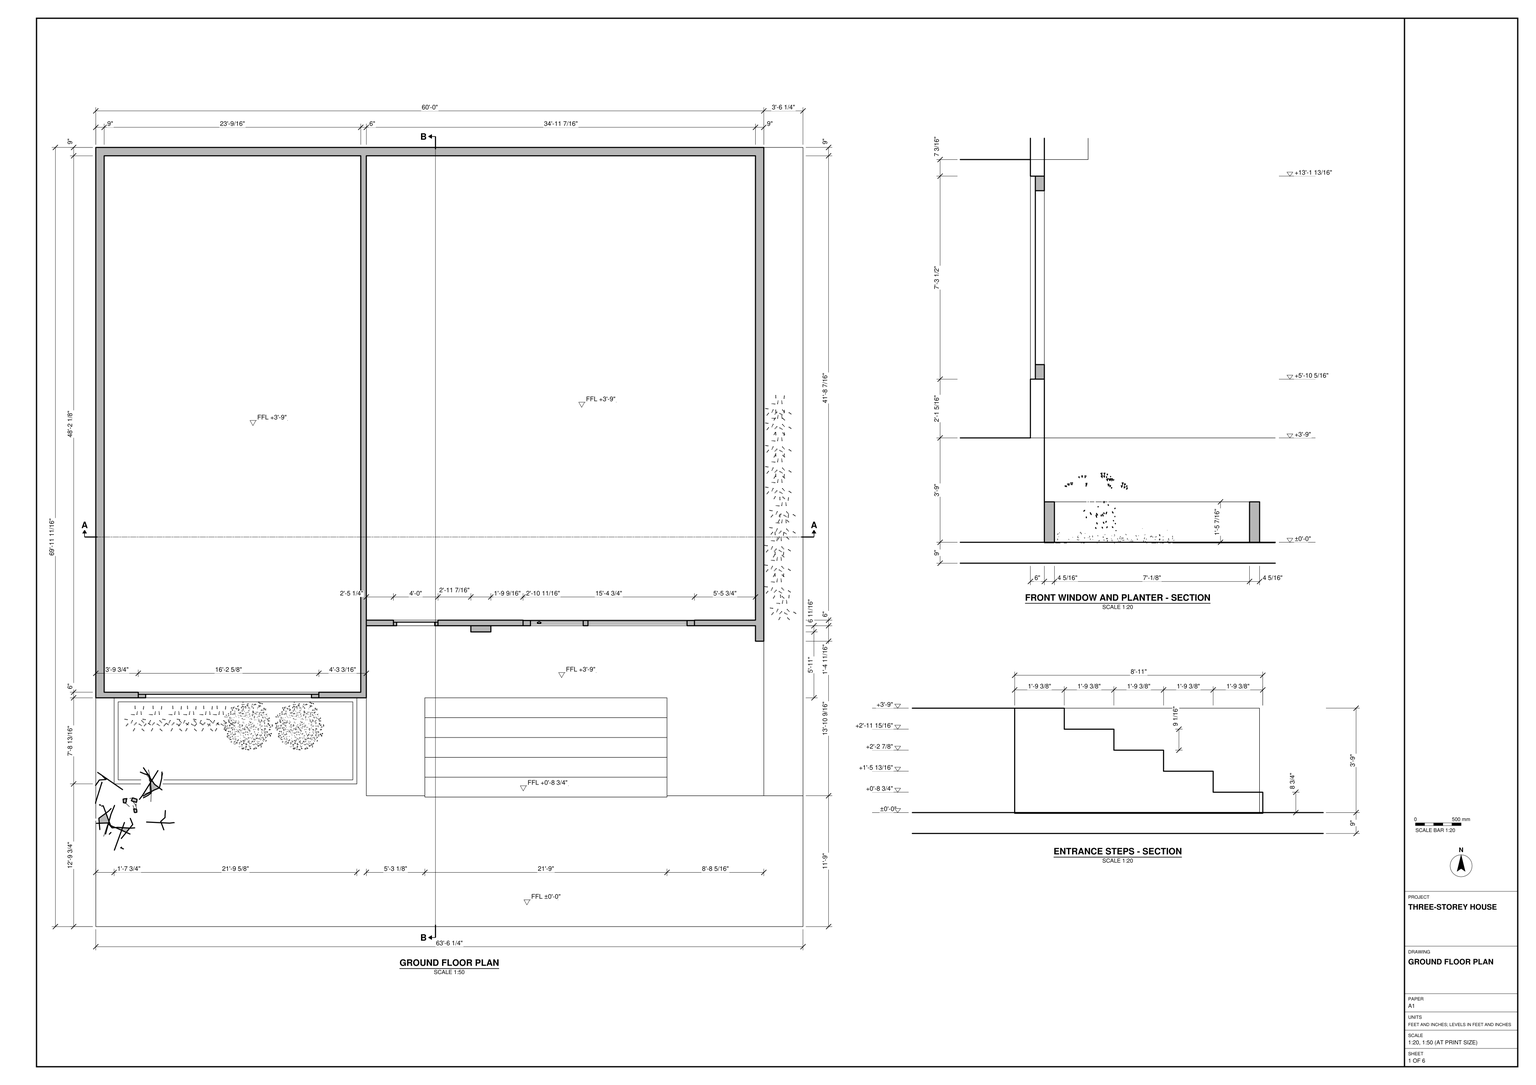
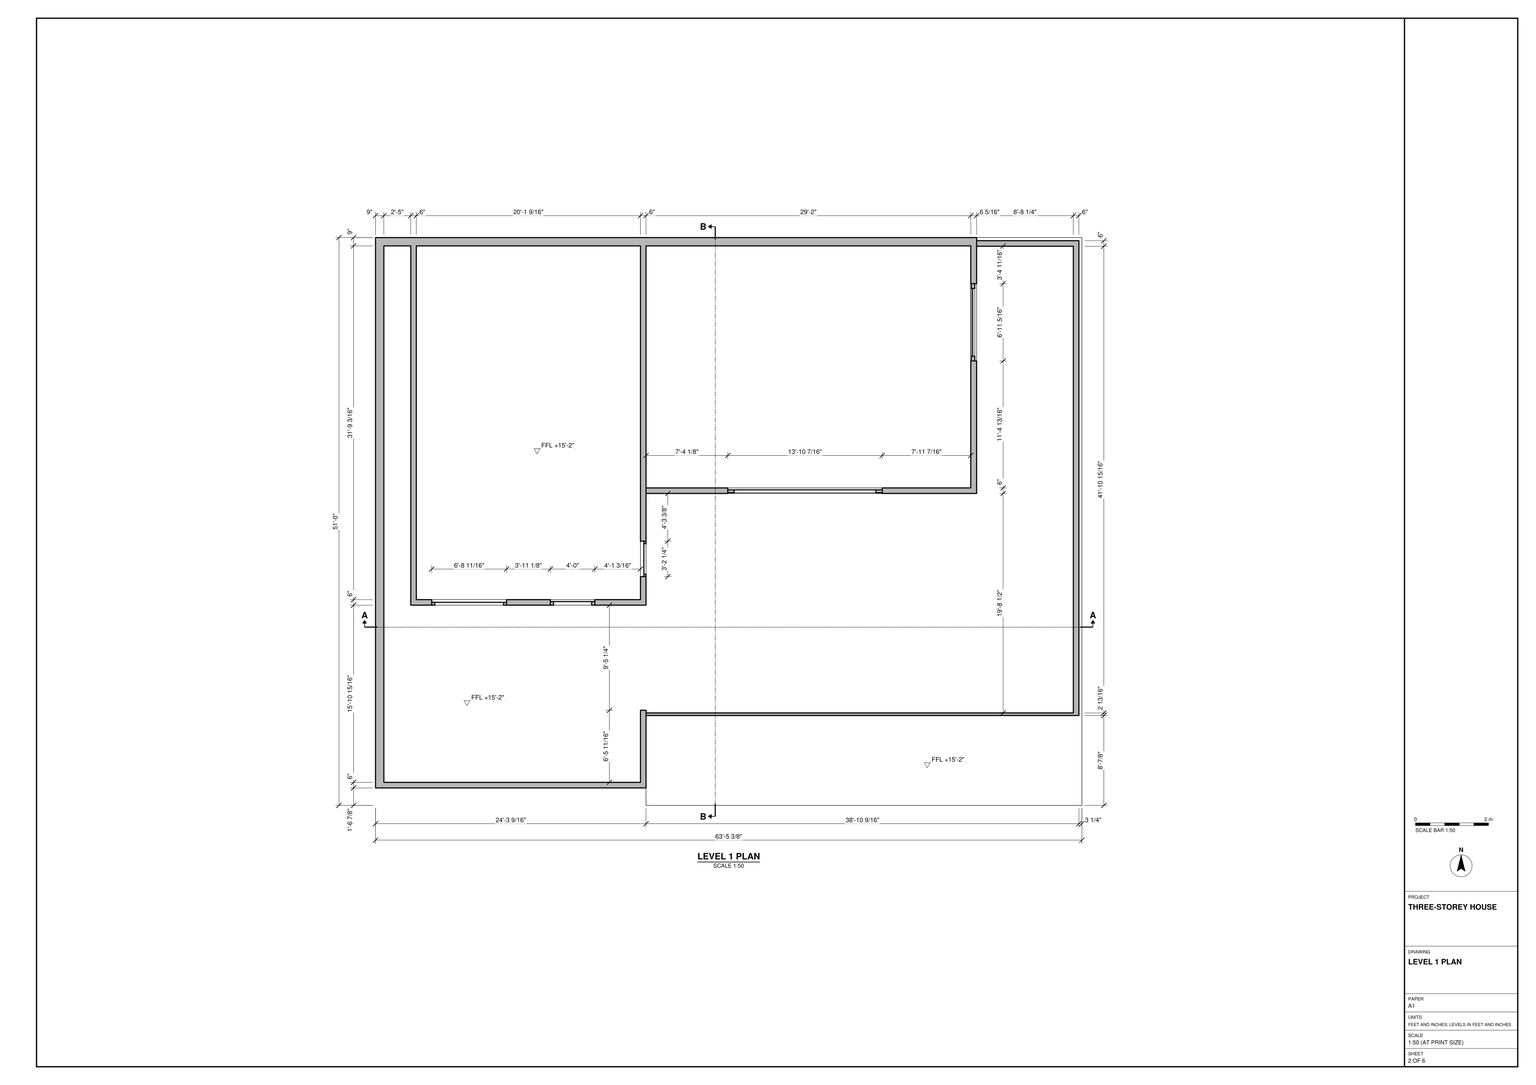
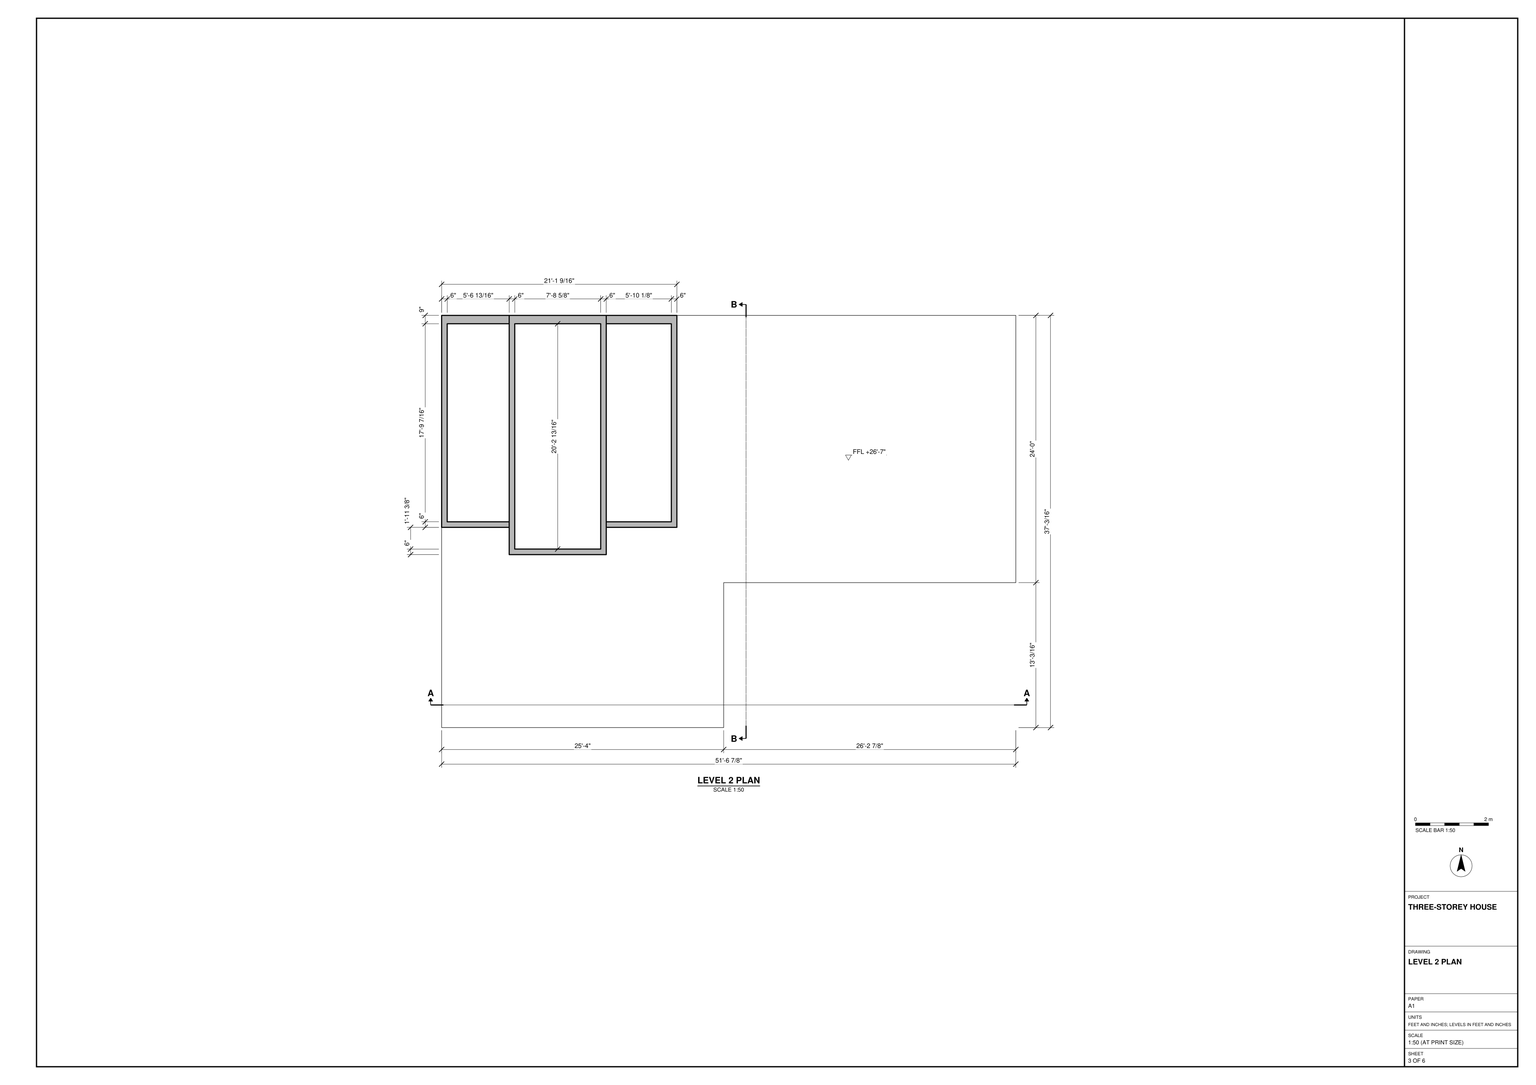
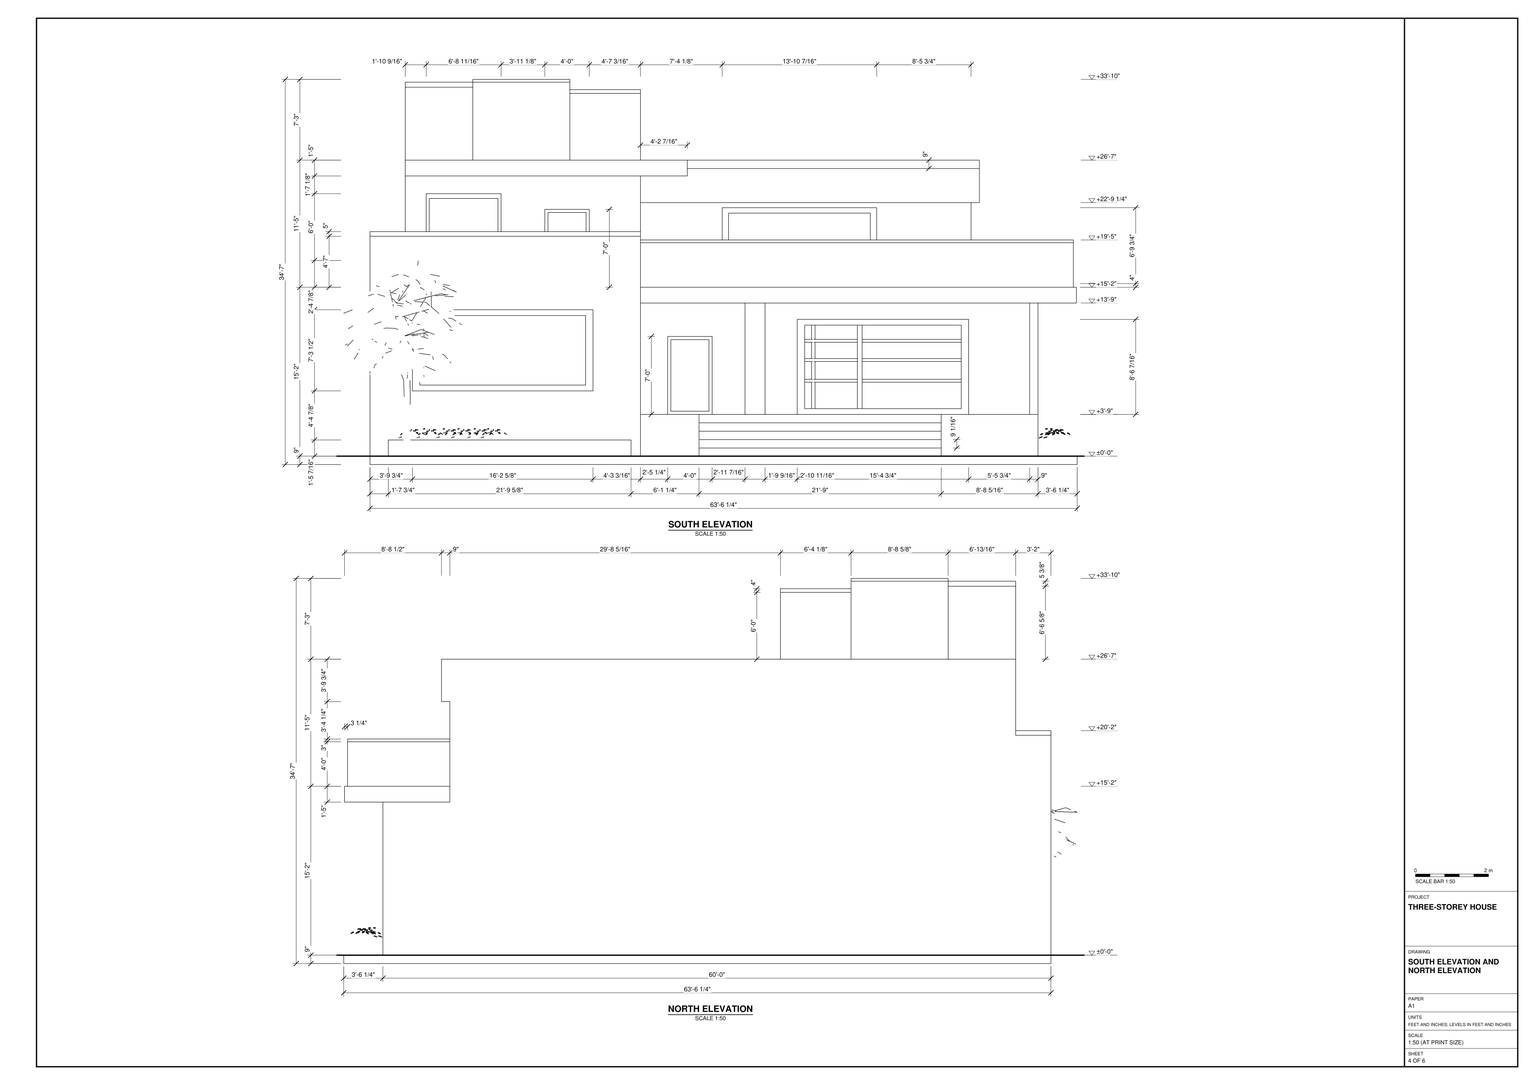
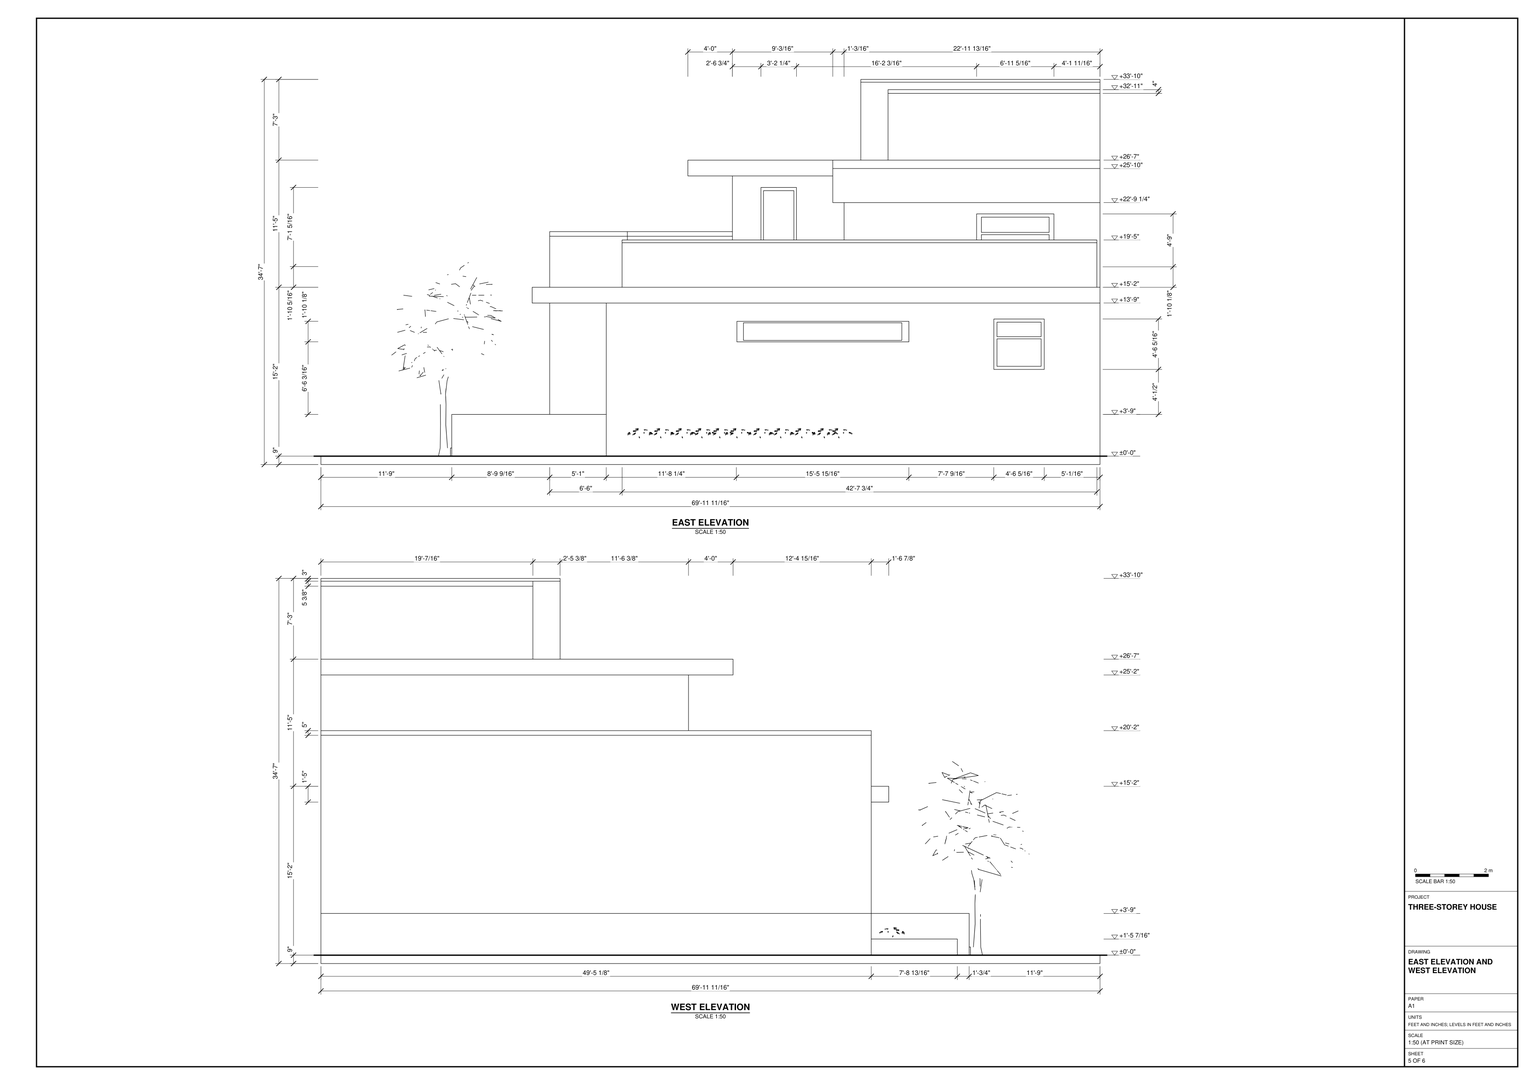
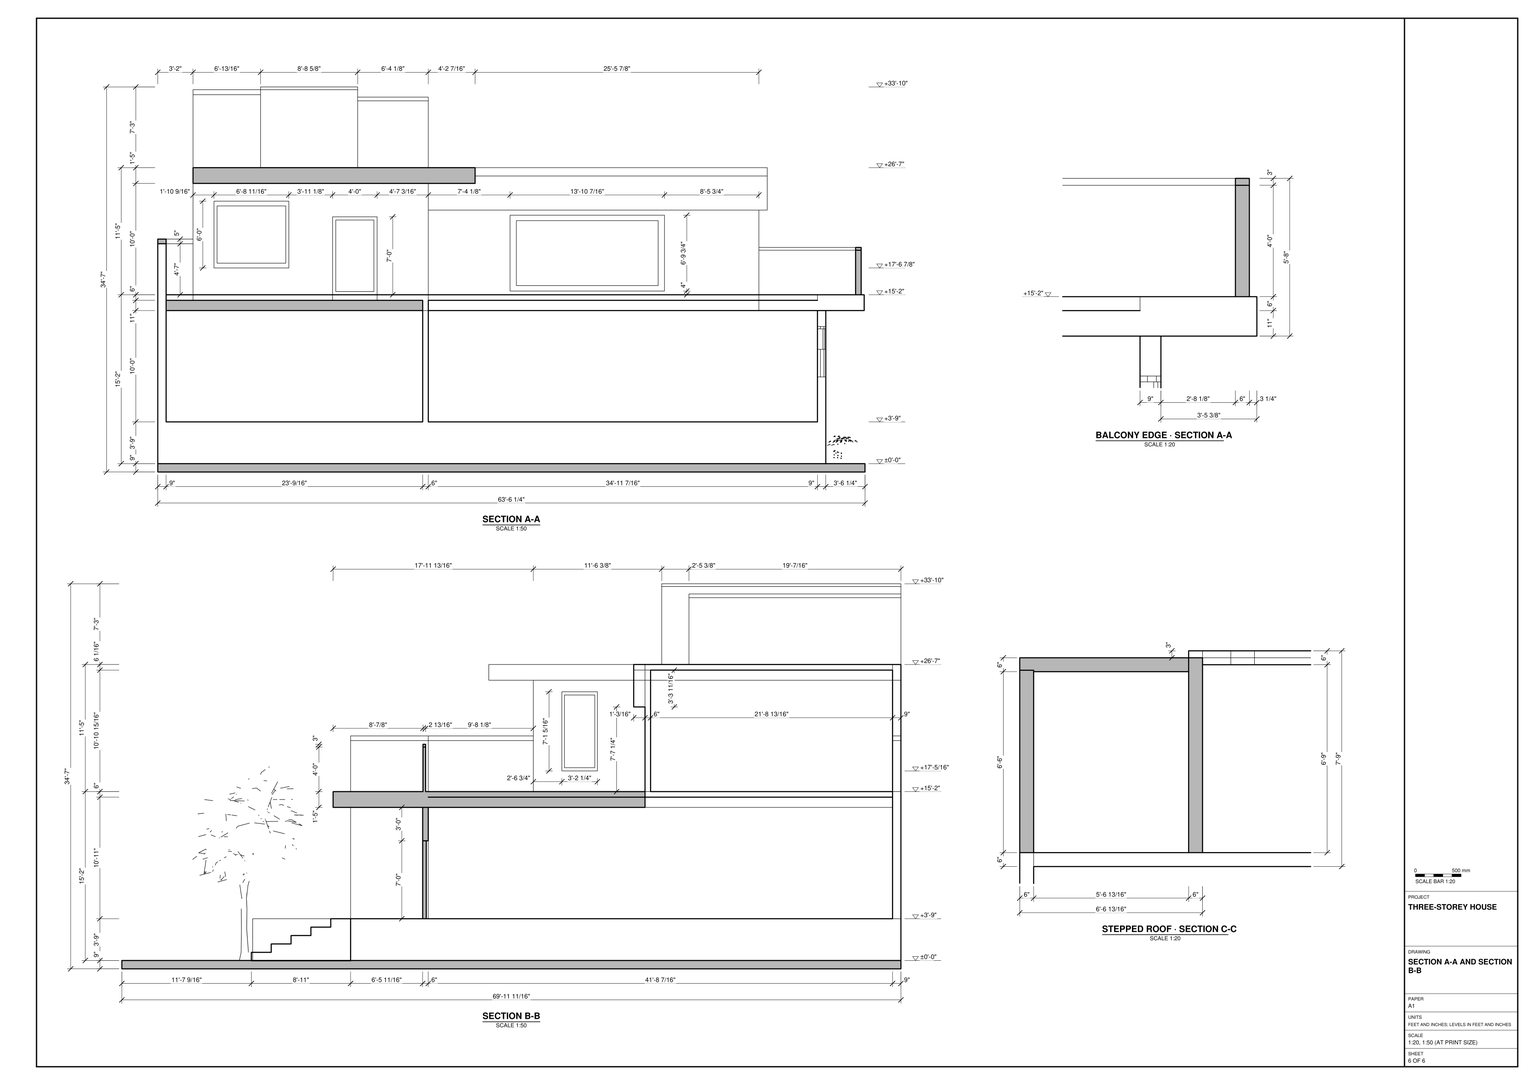
Build the house and its immediate site in SketchUp from task_files/diagram_01.pdf. Work in feet and inches. The complete model measures 66'-1/4" along x, 69'-11 11/16" along y and 34'-7" along z. Use ±0'-0" as the ground datum, with Level 1 at +15'-2" and Level 2 at +26'-7". The ground-floor rooms and entrance landing are raised above the datum to +3'-9".

Lay out the ground floor with the narrower left bay projecting toward the front and the wider right bay set back behind the landing. Form the walls at the thicknesses drawn, including the 9" rear wall and 6" dividing wall. Model the door and window openings in their indicated positions. Use the entrance section for the broad flight of steps and the window section for the low planter beneath the front window. Include the forecourt and planting in the locations shown.

Follow each upper plan separately: set the Level 1 rooms back from the terrace edges and place the three narrow bays at the rear left of Level 2, with the middle bay projecting farther forward. Match the floor and roof slab outlines to the changes in footprint. Keep shell elements such as walls, slabs and roof, and any furniture or joinery pieces shown, in separate groups or components; use components for repeated parts. Plants, decor and loose items may be any suitable library components. Save one SketchUp model as output_files/terraced_three_storey_house_with_entrance_steps.skp.

# SketchUp Ruby script. Lengths in inches.
U = 1.inch
M = Sketchup.active_model
def pt(a) = Geom::Point3d.new(a.map { |v| v * U })
def face(e, loops, mat)
  f = e.add_face(loops[0].map { |a| pt(a) })
  loops[1..].each { |l| e.add_face(l.map { |a| pt(a) }).erase! }
  f.material = f.back_material = mat if mat
  f
end
# faces: each face lists its corners as indices into pts; further lists are holes
def faces(e, pts, list, mat = nil) = list.each { |f| face(e, (f[0].is_a?(Array) ? f : [f]).map { |l| l.map { |i| pts[i] } }, mat) }
# xy, xz, yz: faces in a plane at the given z, y or x. An outline is a flat list of corners, or four numbers for a rectangle; further outlines are holes
def ring(l) = l.size == 4 ? [[l[0], l[1]], [l[2], l[1]], [l[2], l[3]], [l[0], l[3]]] : l.each_slice(2).to_a
def flat(e, list, mat, &to3) = list.each { |f| face(e, (f[0].is_a?(Array) ? f : [f]).map { |l| ring(l).map { |u, v| to3.(u, v) } }, mat) }
def xy(e, z, list, mat = nil) = flat(e, list, mat) { |x, y| [x, y, z] }
def xz(e, y, list, mat = nil) = flat(e, list, mat) { |x, z| [x, y, z] }
def yz(e, x, list, mat = nil) = flat(e, list, mat) { |y, z| [x, y, z] }
def lines(e, pts, list) = list.each { |a, b| e.add_line(pt(pts[a]), pt(pts[b])) }
# prism: a flat outline (further loops are holes) pulled along v
def prism(e, loops, v, mat = nil)
  f = face(e, loops, mat); d = Geom::Vector3d.new(v.map { |x| x * U })
  f.pushpull(f.normal.samedirection?(d) ? d.length : -d.length)
end
def box(e, o, s, mat = nil) = prism(e, [[o, [o[0] + s[0], o[1], o[2]], [o[0] + s[0], o[1] + s[1], o[2]], [o[0], o[1] + s[1], o[2]]]], [0, 0, s[2]], mat)
def at(x, y, z, deg = 0) = Geom::Transformation.translation(pt([x, y, z])) * Geom::Transformation.rotation(ORIGIN, Z_AXIS, deg.degrees)
def axes(o, x, y, z) = Geom::Transformation.new([*x, 0, *y, 0, *z, 0, *pt(o).to_a, 1])
def part(name) = M.definitions.add(name)
# library, detail: a bought-in or finely detailed component or shape, given as its bounding box
def library(name, o, s) = part(name).tap { |d| box(d.entities, o, s) }
def detail(e, o, s) = box(e.add_group.entities, o, s)
def put(e, d, t, mat = nil) = e.add_instance(d, t).tap { |i| i.material = mat if mat }
def group(e, t, mat = nil) = e.add_group.tap { |g| g.transformation = t; g.material = mat if mat }.entities
root = M.entities
M.materials.add("[0047_Khaki]").color = [240, 230, 140]
M.materials.add("[0049_Beige]").color = [245, 245, 220]
M.materials.add("[0062_YellowGreen]").color = [154, 205, 50]
M.materials.add("[0072_DarkSeaGreen]").color = [174, 188, 143]
M.materials.add("[0072_DarkSeaGreen]1").color = [143, 188, 143]
M.materials.add("[0081_CadetBlue]").color = [95, 158, 160]
M.materials.add("[0089_PaleTurquoise]").color = [175, 238, 238]
M.materials.add("[0118_Thistle]").color = [216, 191, 216]
M.materials.add("[0133_Gray]").color = [128, 128, 128]
M.materials.add("[Color C08]").color = [102, 51, 0]
M.materials.add("[Color D02]").color = [255, 229, 153]
M.materials.add("[Color M03]").color = [170, 170, 170]
M.materials.add("[Color_A01]").color = [255, 0, 0]
M.materials.add("[Color_G18]").color = [40, 102, 40]
M.materials.add("[Concrete Block Retaining Gray]").color = [121, 121, 121]
M.materials.add("[Grass Dark Green]").color = [106, 157, 55]
M.materials.add("[Grass Light Green]").color = [138, 158, 69]
M.materials.add("[Pavers with Grass Brick]").color = [187, 192, 176]
M.materials.add("[Stone Vein Gray]").color = [166, 165, 165]
M.materials.add("[Translucent Glass Gray]").color = [128, 128, 128]
M.materials["[Translucent Glass Gray]"].alpha = 0.5
c1 = library("Linden tree",[-68.5,-59.07,-3.48],[128.92,127.11,210.56])
c2 = part("Crocosmia stalk")
xz(c2.entities,0,[[29.25,0,24.47,46.82,16.79,93.27,16.37,94.83,15.75,96.34,14.93,97.74,14.1,98.81,13.27,99.04,12.46,99.23,11.65,99.37,10.82,99.48,9.99,99.54,9.16,99.56,8.33,99.54,7.51,99.48,6.68,99.37,5.86,99.23,5.05,99.04,4.23,98.81,0,98.16,4.09,99.3125,4.92,99.55,5.76,99.74,6.6,99.89,7.45,100,8.31,100.0625,9.16,100.08,10.02,100.0625,10.875,100,11.72,99.89,12.57,99.74,13.4,99.55,14.24,99.3125,15.28,97.98,16.125,96.52,16.77,94.97,17.2,93.36,24.88,46.88,29.67,0.04]],"[Color_G18]")
c3 = part("Group\#7")
xz(c3.entities,0,[[1.6,0,0,2.3,1.58,2.8],[11.99,0,11.82,4.67,14.48,3.96],[6.79,0.79,5.69,4.36,7.9,4.36]])
c4 = part("Crocosmia flower")
put(c4.entities,c3,axes([5.98,1.21,2.14],[1,0,0],[0,0.98769,-0.15643],[0,0.15643,0.98769]))
g1 = group(c4.entities,at(0,1.21,0))
xz(g1,0,[[-3.52,-0.77,3.66,0.34,7.76,1.5,8.59,1.74,9.41,1.92,10.25,2.07,11.08,2.18,11.93,2.24,12.77,2.26,13.62,2.24,14.46,2.18,15.3,2.07,16.13,1.92,16.96,1.74,18,1.44,18.24,2.3,17.18,2.6,16.3125,2.8,15.43,2.95,14.55,3.0625,13.66,3.13,12.77,3.15,11.88,3.13,11,3.0625,10.11,2.95,9.24,2.8,8.37,2.6,7.52,2.36]])
put(c4.entities,c3,axes([5.98,1.21,2.14],[1,0,0],[0,0.96593,0.25882],[0,-0.25882,0.96593]))
c5 = part("Group\#9")
put(c5.entities,c2,at(7.13,1.21,0))
put(c5.entities,c4,at(3.52,0,97.99),"[Color_A01]")
c6 = part("Group\#8")
put(c6.entities,c2,at(7.13,1.21,0))
put(c6.entities,c4,at(3.52,0,97.99),"[Color_A01]")
c7 = part("Group\#10")
put(c7.entities,c5,axes([33.09,14.34,-12.1875],[0.94029,0.03558,0.33851],[0,0.99452,-0.10453],[-0.34038,0.09829,0.93514]))
put(c7.entities,c6,axes([25.49,6.94,1.27],[1,0,0],[0,0.9978,0.06627],[0,-0.06627,0.9978]))
c8 = part("Group\#12")
put(c8.entities,c5,axes([33.09,14.34,-12.1875],[0.94029,0.03558,0.33851],[0,0.99452,-0.10453],[-0.34038,0.09829,0.93514]))
put(c8.entities,c6,axes([25.49,6.94,1.26],[1,0,0],[0,0.9978,0.07356],[0,-0.06627,1.10756]))
c9 = part("Linear leaf")
xy(c9.entities,0,[[0.79,0,0.58,0.87,0.41,1.76,0.29,2.66,0.22,3.58,0.1875,4.5,0.2,5.43,0.26,6.35,0.29,6.57,1.17,6.16,1.18,5.28,1.17,4.39,1.14,3.51,1.08,2.625,1.01,1.75,0.91,0.87],[1.17,6.16,0.29,6.57,0.93,7.17,1.8,7.9375,2.7,8.6875,3.64,9.42,4.59,10.12,3.95,9.33,3.29,8.53,2.61,7.74,1.9,6.95]],"[0062_YellowGreen]")
c10 = part("Group\#22")
put(c10.entities,c9,axes([3.09,18.2,0.54],[1.30643,-1.30643,-0.68344],[1.20815,-1.20815,4.61892],[0.70711,0.70711,0]))
put(c10.entities,c9,axes([3.54,24.84,1.29],[1.05445,-1.05445,-1.28719],[2.27545,-2.27545,3.72805],[0.70711,0.70711,0]))
put(c10.entities,c9,axes([-1.63,23.04,0.27],[2.06861,-2.08759,-0.30686],[0.96675,-0.11843,7.32271],[0.70199,0.70754,-0.08123]))
put(c10.entities,c9,axes([-1.63,22.91,0.84],[2.06861,-1.95964,-0.7823],[0.96675,-1.81223,7.09591],[0.70199,0.70711,0.08495]))
c11 = part("Group\#16")
put(c11.entities,c9,axes([142.1,5.81,0.54],[1.30643,1.30643,-0.68344],[1.20815,1.20815,4.61892],[0.70711,-0.70711,0]))
put(c11.entities,c9,axes([137.375,1.1,0.84],[2.06861,1.95964,-0.7823],[0.96675,1.81223,7.09591],[0.70199,-0.70711,0.08495]))
put(c11.entities,c9,axes([142.55,-0.83,1.29],[1.05445,1.05445,-1.28719],[2.27545,2.27545,3.72805],[0.70711,-0.70711,0]))
put(c11.entities,c9,axes([137.375,0.97,0.27],[2.06861,2.08759,-0.30686],[0.96675,0.11843,7.32271],[0.70199,-0.70754,-0.08123]))
c12 = part("Crocosmia ")
g2 = group(c12.entities,at(0,0,0))
g3 = group(g2,at(0,0,0))
g4 = group(g3,at(13.04,31.23,0.5625))
put(g4,c7,axes([3.46,-0.55,0],[-0.03723,-0.23246,0],[0.23246,-0.03723,0],[0,0,0.23634]))
put(g4,c7,axes([5.71,-0.44,0],[0.0242,-0.23418,0],[-0.23418,-0.0242,0],[0,0,0.23634]))
g5 = group(g3,at(30.75,6.89,0.5625))
put(g5,c7,axes([-2.54,-2.41,0],[-0.16206,0.17077,0],[-0.17077,-0.16206,0],[0,0,0.23634]))
g6 = group(g5,at(-3.82,-4.27,0))
put(g6,c5,axes([-5.12,7.06,-3.25],[-0.18049,0.11942,0.09302],[0.12031,0.20087,-0.02463],[0.0915,-0.02854,0.21587]))
put(g6,c6,axes([-4.26,4.53,0.3],[-0.20073,0.12301,0],[0.12274,0.20029,0.01566],[-0.00774,-0.01264,0.22403]))
g7 = group(g3,at(9.39,-0.8,0.42))
put(g7,c7,axes([-2.625,2.3125,0],[0.15569,0.17659,0],[-0.17659,0.15569,0],[0,0,0.22453]))
put(g7,c8,axes([-4.59,3.42,0],[0.10468,0.21087,0],[0.21087,-0.10468,0],[0,0,0.22453]))
put(g7,c8,axes([-8.77,21.23,-0.42],[0.23414,-0.02461,0],[-0.02461,-0.23414,0],[0,0,0.19085]))
g8 = group(g2,at(5.7,6.33,0.8125))
put(g8,c10,axes([13.91,12.89,0.5],[-0.14417,0.14417,-0.11817],[-0.16647,-0.16647,0],[-0.07042,0.07042,0.17316]),"[0062_YellowGreen]")
put(g8,c10,axes([11.46,2.69,0.5],[0.20214,0.02661,-0.11817],[-0.03073,0.23341,0],[0.09873,0.013,0.17316]),"[0062_YellowGreen]")
g9 = group(g8,at(4.33,8.63,0.49),"[0062_YellowGreen]")
put(g9,c9,axes([4.16,-1.22,-0.3],[-0.33313,-0.174,-0.24196],[-0.35858,-0.54456,0.44909],[0.14623,-0.16466,-0.08356]))
put(g9,c9,axes([5.69,-1.57,-0.25],[-0.2618,-0.0867,-0.28954],[-0.62753,-0.66242,0.20881],[0.14623,-0.16466,-0.08356]))
put(g9,c9,axes([5.42,-0.4,0.22],[-0.53978,-0.33472,-0.27827],[-0.11395,-0.65189,0.69271],[0.14714,-0.15854,-0.09191]))
put(g9,c9,axes([5.38,-0.4375,0.3],[-0.50493,-0.30077,-0.34469],[-0.51698,-0.65817,0.79501],[0.14555,-0.16983,-0.07207]))
put(g8,c10,axes([13.55,3.62,0.5],[0.17657,0.10194,-0.11817],[-0.11771,0.20388,0],[0.08624,0.04979,0.17316]),"[0062_YellowGreen]")
put(g8,c10,axes([11.91,13.98,0.5],[-0.18836,0.07802,-0.11817],[-0.09009,-0.2175,0],[-0.092,0.03811,0.17316]),"[0062_YellowGreen]")
g10 = group(g8,at(8.99,2.63,0.27),"[0062_YellowGreen]")
put(g10,c9,axes([1.79,3.96,0.11],[0.1664,-0.34841,-0.24311],[0.4579,-0.45754,0.77052],[0.19574,0.12348,-0.04333]))
put(g10,c9,axes([2.32,5.43,0.3],[0.09172,-0.26225,-0.33565],[0.57459,-0.7336,0.50887],[0.19574,0.12348,-0.04333]))
put(g10,c9,axes([1.03,5.32,0.47],[0.30723,-0.57597,-0.23823],[0.62693,-0.26669,1.31489],[0.18995,0.12595,-0.05835]))
put(g10,c9,axes([1.125,5.19,0.55],[0.20356,-0.4337,-0.28877],[0.48116,-0.56339,1.27039],[0.15716,0.10279,-0.01678]))
g11 = group(g8,at(15.51,11.18,0.49),"[0062_YellowGreen]")
put(g11,c9,axes([-4.34,-1.06,-0.29],[0.21187,0.31633,-0.25652],[0.02584,0.70318,0.53564],[-0.21414,0.06891,-0.0844]))
put(g11,c9,axes([-5.89,-1.53,-0.23],[0.19483,0.19779,-0.31531],[0.20969,0.9356,0.27713],[-0.21414,0.06891,-0.0844]))
put(g11,c9,axes([-5.04,-2.43,0.23],[0.31461,0.56327,-0.29206],[-0.28686,0.76758,0.96241],[-0.2112,0.06154,-0.09574]))
put(g11,c9,axes([-5.03,-2.37,0.32],[0.30135,0.51422,-0.36204],[0.09995,0.90702,0.92903],[-0.21648,0.07458,-0.07128]))
g12 = group(g8,at(9.18,2.63,0.5),"[0062_YellowGreen]")
put(g12,c9,axes([1.77,3.96,-0.27],[0.11194,-0.34841,-0.27273],[0.60861,-0.45754,0.65704],[0.18234,0.12348,-0.08356]))
put(g12,c9,axes([2.33,5.43,-0.2],[0.01959,-0.26225,-0.34749],[0.66808,-0.7336,0.37665],[0.18234,0.12348,-0.08356]))
put(g12,c9,axes([1.11,5.32,0.24],[0.25067,-0.57597,-0.29759],[0.88756,-0.26669,1.15375],[0.17355,0.12595,-0.09702]))
put(g12,c9,axes([1.16,5.27,0.34],[0.21273,-0.53462,-0.37991],[0.76253,-0.64601,1.11448],[0.1895,0.12157,-0.06825]))
g13 = group(g8,at(4.87,10.84,0.5),"[0062_YellowGreen]")
put(g13,c9,axes([3.37,-2.74,-0.27],[-0.36551,-0.01795,-0.27273],[-0.59947,-0.46946,0.65704],[0.07208,-0.20809,-0.08356]))
put(g13,c9,axes([4.64,-3.66,-0.2],[-0.25839,0.04895,-0.34749],[-0.88152,-0.45544,0.37665],[0.07208,-0.20809,-0.08356]))
put(g13,c9,axes([4.85,-2.45,0.24],[-0.62122,-0.09305,-0.29759],[-0.48731,-0.78829,1.15375],[0.07674,-0.20023,-0.09702]))
put(g13,c9,axes([4.62,-2.79,0.13],[-0.51664,0.02786,-0.31636],[-0.79574,-0.52497,1.14418],[0.08698,-0.18228,-0.04668]))
g14 = group(g2,at(7.45,6.03,0.57),"[0062_YellowGreen]")
put(g14,c11,axes([4.2,-23.18,0],[0.03646,0.23258,0],[-0.23258,0.03646,0],[0,0,0.23634]))
put(g14,c11,axes([22.18,37.74,0],[-0.10588,-0.21027,0],[0.21027,-0.10588,0],[0,0,0.23634]))
put(g14,c11,axes([39.25,-0.41,0.01],[-0.22413,0.07204,0],[-0.07204,-0.22413,0],[0,0,0.26707]))
put(g14,c11,axes([-23.72,7.92,0],[0.23543,0,0],[0,0.23543,0],[0,0,0.23634]))
c13 = library("V-Ray Ready Large Grass Patch",[-29.18,-30.59,-1.91],[60.68,61.32,12.28])
c14 = part("Group\#3")
xy(c14.entities,0,[[0,0,48,3.875]],"[Color C08]")
xy(c14.entities,3.44,[[3.44,0,44.56,3.875]],"[Color C08]")
xy(c14.entities,80.56,[[3.44,0,44.56,3.875]],"[Color C08]")
xy(c14.entities,84,[[0,0,48,3.875]],"[Color C08]")
xz(c14.entities,0,[[[0,0,48,84],[3.44,3.44,44.56,80.56]]],"[Color C08]")
xz(c14.entities,3.875,[[[0,0,48,84],[3.44,3.44,44.56,80.56]]],"[Color C08]")
xz(c14.entities,3.875,[[3.44,3.44,44.56,80.56]],"[Translucent Glass Gray]")
yz(c14.entities,0,[[0,0,3.875,84]],"[Color C08]")
yz(c14.entities,3.44,[[0,3.44,3.875,80.56]],"[Color C08]")
yz(c14.entities,44.56,[[0,3.44,3.875,80.56]],"[Color C08]")
yz(c14.entities,48,[[0,0,3.875,84]],"[Color C08]")
c15 = library("Group\#4",[0,0,0],[91.75,5.625,65.3125])
c16 = part("Group\#1")
xy(c16.entities,0,[[0,0,17.625,207.4375]])
xy(c16.entities,12.83,[[0,12.83,7.125,194.61],[7.125,12.83,17.625,194.61]],"[Color C08]")
xy(c16.entities,125.93,[[0,12.83,7.125,194.61],[7.125,12.83,17.625,194.61]])
xy(c16.entities,134.79,[[0,12.83,7.125,194.61],[7.125,12.83,17.625,194.61]],"[Color C08]")
xy(c16.entities,194.61,[[0,12.83,7.125,194.61],[7.125,12.83,17.625,194.61]])
xy(c16.entities,207.4375,[[0,0,17.625,207.4375]],"[Color C08]")
xz(c16.entities,0,[[0,0,17.625,207.4375]],"[Color C08]")
xz(c16.entities,12.83,[[0,12.83,7.125,125.93],[7.125,12.83,17.625,125.93],[0,134.79,7.125,194.61],[7.125,134.79,17.625,194.61]],"[Color C08]")
xz(c16.entities,194.61,[[0,12.83,7.125,125.93],[7.125,12.83,17.625,125.93],[0,134.79,7.125,194.61],[7.125,134.79,17.625,194.61]],"[Color C08]")
xz(c16.entities,207.4375,[[0,0,17.625,207.4375]],"[Color C08]")
yz(c16.entities,0,[[[0,0,207.4375,207.4375],[12.83,12.83,194.61,125.93],[12.83,134.79,194.61,194.61]]],"[Color C08]")
yz(c16.entities,7.125,[[12.83,12.83,194.61,125.93],[12.83,134.79,194.61,194.61]],"[Translucent Glass Gray]")
yz(c16.entities,17.625,[[[0,0,207.4375,207.4375],[12.83,12.83,194.61,125.93],[12.83,134.79,194.61,194.61]]],"[Color C08]")
xy(root,-45,[[0,0,762.25,839.6875]])
xy(root,-36,[[291.5625,141,354.66,141,354.66,246.5625,615.66,246.5625,615.66,141,720,141,720,839.6875,0,839.6875,0,246.5625,291.5625,246.5625]])
xy(root,-36,[[[19.76,153.75,281.39,246.5625],[24.11,158.09,277.04,242.22]]],"[Concrete Block Retaining Gray]")
xy(root,-36,[[720,141,762.25,839.6875]],"[Grass Dark Green]")
xy(root,-36,[[24.11,158.09,277.04,242.22]],"[Grass Light Green]")
xy(root,-36,[[0,0,762.25,0,762.25,141,615.66,141,615.66,246.5625,354.66,246.5625,354.66,141,291.5625,141,291.5625,246.5625,281.39,246.5625,281.39,153.75,19.76,153.75,19.76,246.5625,0,246.5625]],"[Pavers with Grass Brick]")
xy(root,-18.5625,[[[19.76,153.75,281.39,246.5625],[24.11,158.09,277.04,242.22]]],"[Concrete Block Retaining Gray]")
xy(root,9,[[9,252.5625,285.5625,830.6875],[404.24,317.5625,425.81,324.25],[291.5625,324.25,320.8,330.25],[368.8,324.25,460.5,330.25],[460.5,324.25,645.25,330.25],
  [291.5625,330.25,711,830.6875]])
xy(root,9,[[291.5625,141,354.66,141,354.66,246.5625,615.66,246.5625,615.66,141,720,141,720,307.5625,711,307.5625,711,324.25,425.81,324.25,425.81,317.5625,404.24,317.5625,404.24,324.25,368.8,324.25,368.8,330.25,320.8,330.25,320.8,324.25,291.5625,324.25]],"[0049_Beige]")
xy(root,34.34,[[45.77,246.5625,240.39,252.5625]])
xy(root,57.48,[[711,725.28,720,779.6]])
xy(root,87.17,[[711,448.34,720,633.72]])
xy(root,93,[[320.8,324.25,368.8,330.25]])
xy(root,109.3,[[711,448.34,720,633.72]])
xy(root,111.43,[[460.5,324.25,645.25,330.25]])
xy(root,111.79,[[711,725.28,720,779.6]])
xy(root,121.84,[[45.77,246.5625,240.39,252.5625]])
xy(root,129,[[9,252.5625,9,830.6875,38,830.6875,38,443.5,188.4,443.5,188.4,449.5,236.4,449.5,236.4,443.5,285.5625,443.5,285.5625,252.5625],[711,307.5625,711,324.25,291.5625,324.25,291.5625,330.25,720,330.25,720,307.5625],[404.24,317.5625,425.81,324.25],[291.5625,330.25,291.5625,563.875,647.875,563.875,647.875,830.6875,711,830.6875,711,330.25],[711,330.25,720,839.6875],
  [647.875,830.6875,711,839.6875]])
xy(root,129,[[291.5625,227.6875,291.5625,324.25,404.24,324.25,404.24,317.5625,425.81,317.5625,425.81,324.25,711,324.25,711,307.5625,720,307.5625,720,839.6875,761.375,839.6875,761.375,227.6875]],"[0072_DarkSeaGreen]1")
xy(root,140,[[9,252.5625,285.5625,830.6875],[291.5625,330.25,711,830.6875]])
xy(root,146,[[752.125,324.5625,752.125,830.3125,647.875,830.3125,647.875,836.3125,758.125,836.3125,758.125,324.5625],[44,449.5,285.5625,830.6875],[291.5625,569.875,641.5625,830.6875]])
xy(root,146,[[291.5625,227.6875,761.375,227.6875,761.375,839.6875,647.875,839.6875,647.875,836.3125,758.125,836.3125,758.125,324.5625,291.5625,324.5625]],"[0072_DarkSeaGreen]1")
xy(root,146,[[9,252.5625,285.5625,252.5625,285.5625,330.25,291.5625,330.25,291.5625,327.375,752.125,327.375,752.125,830.3125,647.875,830.3125,647.875,563.875,291.5625,563.875,291.5625,443.5,236.4,443.5,236.4,449.5,188.4,449.5,188.4,443.5,38,443.5,38,830.6875,9,830.6875]],"[Stone Vein Gray]")
xy(root,150.02,[[379.68,563.875,546.12,569.875]])
xy(root,168.11,[[641.5625,706.7,647.875,790.02]])
xy(root,168.29,[[285.5625,474.26,291.5625,512.51]])
xy(root,174.9,[[60.59,443.5,141.27,449.5]])
xy(root,194,[[291.5625,324.5625,291.5625,327.375,752.125,327.375,752.125,830.3125,647.875,830.3125,647.875,836.3125,758.125,836.3125,758.125,324.5625]])
xy(root,197,[[291.5625,324.5625,758.125,324.5625,758.125,836.3125,647.875,836.3125,647.875,830.3125,752.125,830.3125,752.125,327.375,291.5625,327.375]],"[Color D02]")
xy(root,201,[[0,246.5625,0,839.6875,9,839.6875,9,252.5625,285.5625,252.5625,285.5625,330.25,291.5625,330.25,291.5625,246.5625]])
xy(root,206,[[0,246.5625,291.5625,246.5625,291.5625,330.25,285.5625,330.25,285.5625,252.5625,9,252.5625,9,830.6875,38,830.6875,38,839.6875,0,839.6875]],"[Color D02]")
xy(root,225.11,[[641.5625,706.7,647.875,790.02]])
xy(root,230,[[188.4,443.5,236.4,449.5]])
xy(root,231.77,[[379.68,563.875,546.12,569.875]])
xy(root,237.25,[[291.5625,551.6875,291.5625,563.875,647.875,563.875,647.875,839.6875,656.875,839.6875,656.875,551.6875]])
xy(root,246.9,[[60.59,443.5,141.27,449.5]])
xy(root,253.61,[[285.5625,474.26,291.5625,512.51]])
xy(root,266,[[38,395.5,291.5625,443.5],[291.5625,395.5,342,551.6875],[291.5625,551.6875,342,563.875]])
xy(root,276.9375,[[291.5625,569.875,641.5625,830.6875]])
xy(root,277,[[44,449.5,285.5625,830.6875]])
xy(root,283,[[[110.8125,581.875,215.4375,839.6875],[116.8125,587.875,209.4375,830.6875]],[116.8125,587.875,209.4375,830.6875],[38,611.25,38,839.6875,110.8125,839.6875,110.8125,830.6875,44,830.6875,44,617.25,110.8125,617.25,110.8125,611.25],[215.4375,611.25,215.4375,617.25,285.5625,617.25,285.5625,830.6875,215.4375,830.6875,215.4375,839.6875,291.5625,839.6875,291.5625,611.25],[44,617.25,110.8125,830.6875],
  [215.4375,617.25,285.5625,830.6875]])
xy(root,283,[[38,395.5,342,395.5,342,551.6875,656.875,551.6875,656.875,839.6875,291.5625,839.6875,291.5625,611.25,215.4375,611.25,215.4375,581.875,110.8125,581.875,110.8125,611.25,38,611.25]],"[0133_Gray]")
xy(root,353,[[215.4375,617.25,285.5625,830.6875]])
xy(root,355,[[215.4375,611.25,215.4375,617.25,285.5625,617.25,285.5625,830.6875,215.4375,830.6875,215.4375,839.6875,291.5625,839.6875,291.5625,611.25]])
xy(root,359,[[215.4375,611.25,291.5625,839.6875]],"[0133_Gray]")
xy(root,361,[[44,617.25,110.8125,830.6875]])
xy(root,361.625,[[38,611.25,38,839.6875,110.8125,839.6875,110.8125,830.6875,44,830.6875,44,617.25,110.8125,617.25,110.8125,611.25]])
xy(root,364,[[116.8125,587.875,209.4375,830.6875]])
xy(root,367,[[[110.8125,581.875,215.4375,839.6875],[116.8125,587.875,209.4375,830.6875]]])
xy(root,367,[[38,611.25,110.8125,839.6875]],"[0133_Gray]")
xy(root,370,[[110.8125,581.875,215.4375,839.6875]],"[0133_Gray]")
xz(root,0,[[0,-45,762.25,-36]])
xz(root,141,[[291.5625,-36,354.66,9],[615.66,-36,720,9]],"[0049_Beige]")
xz(root,153.75,[[19.76,-36,281.39,-18.5625]],"[Concrete Block Retaining Gray]")
xz(root,158.09,[[24.11,-36,277.04,-18.5625]],"[Concrete Block Retaining Gray]")
xz(root,227.6875,[[291.5625,129,761.375,146]],"[0072_DarkSeaGreen]1")
xz(root,242.22,[[24.11,-36,277.04,-18.5625]],"[Concrete Block Retaining Gray]")
xz(root,246.5625,[[354.66,-36,615.66,9]])
xz(root,246.5625,[[[0,-36,19.76,-36,19.76,-18.5625,281.39,-18.5625,281.39,-36,291.5625,-36,291.5625,201,0,201],[45.77,34.34,240.39,121.84]]],"[0081_CadetBlue]")
xz(root,246.5625,[[0,201,291.5625,206]],"[Color D02]")
xz(root,246.5625,[[19.76,-36,281.39,-18.5625]],"[Concrete Block Retaining Gray]")
xz(root,252.5625,[[[9,9,285.5625,129],[45.77,34.34,240.39,121.84]],[9,129,285.5625,140],[9,140,285.5625,146]])
xz(root,252.5625,[[9,201,285.5625,206]],"[Color D02]")
xz(root,252.5625,[[9,146,285.5625,201]],"[Color M03]")
xz(root,307.5625,[[711,9,720,129]],"[0118_Thistle]")
xz(root,317.5625,[[404.24,9,425.81,129]],"[0118_Thistle]")
xz(root,324.25,[[404.24,9,425.81,129]])
xz(root,324.25,[[291.5625,9,320.8,9,320.8,93,368.8,93,368.8,9,404.24,9,404.24,129,291.5625,129],[425.81,9,460.5,9,460.5,111.43,645.25,111.43,645.25,9,711,9,711,129,425.81,129]],"[0118_Thistle]")
xz(root,324.5625,[[291.5625,194,758.125,197]],"[Color D02]")
xz(root,324.5625,[[291.5625,146,758.125,194]],"[Translucent Glass Gray]")
xz(root,327.375,[[291.5625,194,752.125,197]],"[Color D02]")
xz(root,327.375,[[291.5625,146,752.125,194]],"[Translucent Glass Gray]")
xz(root,330.25,[[291.5625,9,291.5625,129,711,129,711,9,645.25,9,645.25,111.43,460.5,111.43,460.5,9,368.8,9,368.8,93,320.8,93,320.8,9],[285.5625,129,291.5625,146]])
xz(root,330.25,[[285.5625,201,291.5625,206]],"[0047_Khaki]")
xz(root,330.25,[[285.5625,146,291.5625,201]],"[0081_CadetBlue]")
xz(root,395.5,[[38,266,342,283]],"[0133_Gray]")
xz(root,443.5,[[38,129,188.4,146],[236.4,129,291.5625,146]])
xz(root,443.5,[[[38,146,188.4,146,188.4,230,236.4,230,236.4,146,291.5625,146,291.5625,266,38,266],[60.59,174.9,141.27,246.9]]],"[0089_PaleTurquoise]")
xz(root,448.34,[[711,87.17,720,109.3]])
xz(root,449.5,[[188.4,129,236.4,146],[[44,146,44,266,285.5625,266,285.5625,146,236.4,146,236.4,230,188.4,230,188.4,146],[60.59,174.9,141.27,246.9]],[44,266,285.5625,277]])
xz(root,474.26,[[285.5625,168.29,291.5625,253.61]])
xz(root,512.51,[[285.5625,168.29,291.5625,253.61]])
xz(root,551.6875,[[291.5625,237.25,656.875,237.25,656.875,274,342,274,342,266,291.5625,266]],"[0081_CadetBlue]")
xz(root,551.6875,[[342,274,656.875,283]],"[0133_Gray]")
xz(root,563.875,[[291.5625,129,647.875,146]])
xz(root,563.875,[[[291.5625,146,647.875,237.25],[379.68,150.02,546.12,231.77]]],"[0089_PaleTurquoise]")
xz(root,569.875,[[[291.5625,146,641.5625,266],[379.68,150.02,546.12,231.77]],[291.5625,266,641.5625,276.9375]])
xz(root,581.875,[[110.8125,283,215.4375,367]],"[0081_CadetBlue]")
xz(root,581.875,[[110.8125,367,215.4375,370]],"[0133_Gray]")
xz(root,587.875,[[116.8125,283,209.4375,364],[116.8125,364,209.4375,367]])
xz(root,611.25,[[38,283,110.8125,361.625],[215.4375,283,291.5625,355]],"[0081_CadetBlue]")
xz(root,611.25,[[215.4375,355,291.5625,359],[38,361.625,110.8125,367]],"[0133_Gray]")
xz(root,617.25,[[44,283,110.8125,361],[215.4375,283,285.5625,353],[215.4375,353,285.5625,355],[44,361,110.8125,361.625]])
xz(root,633.72,[[711,87.17,720,109.3]])
xz(root,706.7,[[641.5625,168.11,647.875,225.11]])
xz(root,725.28,[[711,57.48,720,111.79]])
xz(root,779.6,[[711,57.48,720,111.79]])
xz(root,790.02,[[641.5625,168.11,647.875,225.11]])
xz(root,830.3125,[[647.875,194,752.125,197]],"[Color D02]")
xz(root,830.3125,[[647.875,146,752.125,194]],"[Color M03]")
xz(root,830.6875,[[9,9,285.5625,129],[291.5625,9,711,9,711,129,647.875,129,647.875,140,291.5625,140],[9,129,38,140],[38,129,285.5625,140],[9,140,38,146],
  [291.5625,140,356.35,146],[356.35,140,387.41,146],[9,146,38,201],[44,146,285.5625,266],[291.5625,146,641.5625,266],
  [44,266,285.5625,277],[291.5625,266,641.5625,276.9375],[44,283,110.8125,361],[116.8125,283,209.4375,364],[215.4375,283,285.5625,353],
  [215.4375,353,285.5625,355],[44,361,54.52,361.625],[54.52,361,59.77,361.625],[59.77,361,110.8125,361.625],[116.8125,364,129.01,367],
  [129.01,364,139.19,367],[139.19,364,209.4375,367]])
xz(root,830.6875,[[9,201,38,206]],"[Color D02]")
xz(root,836.3125,[[647.875,146,758.125,194]],"[0089_PaleTurquoise]")
xz(root,836.3125,[[647.875,194,758.125,197]],"[Color D02]")
xz(root,839.6875,[[0,-45,762.25,-36]])
xz(root,839.6875,[[647.875,129,761.375,146]],"[0072_DarkSeaGreen]1")
xz(root,839.6875,[[38,283,110.8125,361.625],[110.8125,283,215.4375,367],[215.4375,283,291.5625,355]],"[0081_CadetBlue]")
xz(root,839.6875,[[0,-36,0,201,38,201,38,283,656.875,283,656.875,237.25,647.875,237.25,647.875,129,720,129,720,-36]],"[0089_PaleTurquoise]")
xz(root,839.6875,[[215.4375,355,291.5625,359],[38,361.625,110.8125,367],[110.8125,367,215.4375,370]],"[0133_Gray]")
xz(root,839.6875,[[0,201,38,206]],"[Color D02]")
yz(root,0,[[0,-45,839.6875,-36],[246.5625,-36,839.6875,9]])
yz(root,0,[[246.5625,9,839.6875,201]],"[0081_CadetBlue]")
yz(root,0,[[246.5625,201,839.6875,206]],"[Color D02]")
yz(root,9,[[252.5625,9,830.6875,129],[252.5625,129,259.25,140],[259.25,129,830.6875,140],[252.5625,140,259.25,146],[259.25,140,830.6875,146]])
yz(root,9,[[252.5625,201,830.6875,206]],"[Color D02]")
yz(root,9,[[252.5625,146,830.6875,201]],"[Color M03]")
yz(root,19.76,[[153.75,-36,246.5625,-18.5625]],"[Concrete Block Retaining Gray]")
yz(root,24.11,[[158.09,-36,242.22,-18.5625]],"[Concrete Block Retaining Gray]")
yz(root,38,[[443.5,129,830.6875,146]])
yz(root,38,[[611.25,283,839.6875,361.625]],"[0081_CadetBlue]")
yz(root,38,[[443.5,146,443.5,266,839.6875,266,839.6875,206,830.6875,206,830.6875,146]],"[0089_PaleTurquoise]")
yz(root,38,[[395.5,266,839.6875,283],[611.25,361.625,839.6875,367]],"[0133_Gray]")
yz(root,44,[[449.5,146,830.6875,266],[449.5,266,830.6875,277],[617.25,283,830.6875,361],[617.25,361,830.6875,361.625]])
yz(root,45.77,[[246.5625,34.34,252.5625,121.84]])
yz(root,60.59,[[443.5,174.9,449.5,246.9]])
yz(root,110.8125,[[611.25,283,617.25,361.625],[617.25,283,830.6875,361],[830.6875,283,839.6875,361.625],[617.25,361,830.6875,367],[611.25,361.625,617.25,367],
  [830.6875,361.625,839.6875,367]])
yz(root,110.8125,[[581.875,283,611.25,367]],"[0081_CadetBlue]")
yz(root,110.8125,[[581.875,367,839.6875,370]],"[0133_Gray]")
yz(root,116.8125,[[587.875,283,830.6875,364],[587.875,364,830.6875,367]])
yz(root,141.27,[[443.5,174.9,449.5,246.9]])
yz(root,188.4,[[443.5,129,449.5,146],[443.5,146,449.5,230]])
yz(root,209.4375,[[587.875,283,830.6875,364],[587.875,364,830.6875,367]])
yz(root,215.4375,[[611.25,283,617.25,355],[617.25,283,830.6875,353],[830.6875,283,839.6875,355],[617.25,353,830.6875,359],[611.25,355,617.25,359],
  [830.6875,355,839.6875,359]])
yz(root,215.4375,[[581.875,283,611.25,283,611.25,359,839.6875,359,839.6875,367,581.875,367]],"[0081_CadetBlue]")
yz(root,215.4375,[[581.875,367,839.6875,370]],"[0133_Gray]")
yz(root,236.4,[[443.5,129,449.5,146],[443.5,146,449.5,230]])
yz(root,240.39,[[246.5625,34.34,252.5625,121.84]])
yz(root,277.04,[[158.09,-36,242.22,-18.5625]],"[Concrete Block Retaining Gray]")
yz(root,281.39,[[153.75,-36,246.5625,-18.5625]],"[Concrete Block Retaining Gray]")
yz(root,285.5625,[[252.5625,9,830.6875,129],[252.5625,129,330.25,140],[330.25,129,830.6875,140],[252.5625,140,330.25,146],[252.5625,146,330.25,201],
  [[449.5,146,830.6875,266],[474.26,168.29,512.51,253.61]],[449.5,266,830.6875,277],[617.25,283,830.6875,353],[617.25,353,830.6875,355]])
yz(root,285.5625,[[252.5625,201,330.25,206]],"[Color D02]")
yz(root,291.5625,[[324.25,9,330.25,129],[330.25,9,830.6875,129],[246.5625,129,324.25,146],[324.25,129,330.25,129,330.25,146,327.375,146,327.375,194,324.5625,194,324.5625,146,324.25,146],[330.25,129,443.5,140],
  [443.5,129,563.875,140],[563.875,129,830.6875,140],[443.5,140,563.875,146],[563.875,146,569.875,266],[569.875,146,830.6875,266],
  [324.5625,194,327.375,197],[551.6875,237.25,563.875,266],[569.875,266,830.6875,276.9375]])
yz(root,291.5625,[[141,-36,246.5625,9]],"[0049_Beige]")
yz(root,291.5625,[[227.6875,129,246.5625,146]],"[0072_DarkSeaGreen]1")
yz(root,291.5625,[[246.5625,9,324.25,129],[246.5625,146,324.5625,146,324.5625,197,327.375,197,327.375,146,330.25,146,330.25,201,246.5625,201],[611.25,283,839.6875,355]],"[0081_CadetBlue]")
yz(root,291.5625,[[[443.5,146,563.875,146,563.875,237.25,551.6875,237.25,551.6875,266,443.5,266],[474.26,168.29,512.51,253.61]]],"[0089_PaleTurquoise]")
yz(root,291.5625,[[611.25,355,839.6875,359]],"[0133_Gray]")
yz(root,291.5625,[[246.5625,201,330.25,206]],"[Color D02]")
yz(root,320.8,[[324.25,9,330.25,93]])
yz(root,342,[[395.5,266,551.6875,283]],"[0133_Gray]")
yz(root,354.66,[[141,-36,246.5625,9]],"[0049_Beige]")
yz(root,368.8,[[324.25,9,330.25,93]])
yz(root,379.68,[[563.875,150.02,569.875,231.77]])
yz(root,404.24,[[317.5625,9,324.25,129]],"[0118_Thistle]")
yz(root,425.81,[[317.5625,9,324.25,129]],"[0118_Thistle]")
yz(root,460.5,[[324.25,9,330.25,111.43]])
yz(root,546.12,[[563.875,150.02,569.875,231.77]])
yz(root,615.66,[[141,-36,246.5625,9]],"[0049_Beige]")
yz(root,641.5625,[[[569.875,146,830.6875,276.9375],[706.7,168.11,790.02,225.11]]])
yz(root,645.25,[[324.25,9,330.25,111.43]])
yz(root,647.875,[[563.875,129,830.6875,146],[830.6875,129,839.6875,146],[830.3125,146,830.6875,194],[830.6875,146,836.3125,194],[830.3125,194,830.6875,197],
  [830.6875,194,836.3125,197]])
yz(root,647.875,[[[563.875,146,830.3125,146,830.3125,197,836.3125,197,836.3125,146,839.6875,146,839.6875,237.25,563.875,237.25],[706.7,168.11,790.02,225.11]]],"[0089_PaleTurquoise]")
yz(root,656.875,[[551.6875,237.25,839.6875,274]],"[0081_CadetBlue]")
yz(root,656.875,[[551.6875,274,839.6875,283]],"[0133_Gray]")
yz(root,711,[[[330.25,9,830.6875,129],[448.34,87.17,633.72,109.3],[725.28,57.48,779.6,111.79]]])
yz(root,711,[[307.5625,9,324.25,129]],"[0118_Thistle]")
yz(root,720,[[141,-36,307.5625,9]],"[0049_Beige]")
yz(root,720,[[[307.5625,-36,839.6875,129],[448.34,87.17,633.72,109.3],[725.28,57.48,779.6,111.79]]],"[0118_Thistle]")
yz(root,752.125,[[327.375,194,830.3125,197]],"[Color D02]")
yz(root,752.125,[[327.375,146,830.3125,194]],"[Color M03]")
yz(root,758.125,[[324.5625,146,836.3125,194]],"[0089_PaleTurquoise]")
yz(root,758.125,[[324.5625,194,836.3125,197]],"[Color D02]")
yz(root,761.375,[[227.6875,129,839.6875,146]],"[0072_DarkSeaGreen]1")
yz(root,762.25,[[0,-45,839.6875,-36]])
# 26 loose lines left out
put(root,c1,at(38.5,132.91,-32.52))
put(root,c12,at(725.0625,329.19,-32.8))
put(root,c12,at(719.2,352.27,-32.8))
put(root,c12,at(719.2,375.52,-32.8))
put(root,c12,at(719.2,396.65,-32.8))
put(root,c12,at(724.38,415.9,-32.8))
put(root,c12,at(724.38,434.4,-32.8))
put(root,c12,at(719.93,459.44,-32.8))
put(root,c12,at(719.93,481.57,-32.8))
put(root,c12,at(719.93,504.32,-32.8))
put(root,c12,at(719.93,528.57,-32.8))
put(root,c12,at(719.93,544.19,-32.8))
put(root,c12,at(29.37,209.32,-32.8))
put(root,c12,at(48.81,209.32,-32.8))
put(root,c12,at(70.06,209.32,-32.8))
put(root,c12,at(85.87,209.32,-32.8))
put(root,c12,at(103.37,209.32,-32.8))
put(root,c12,at(117.81,209.32,-32.8))
put(root,c13,at(164.17,217.38,-36))
put(root,c13,at(219.42,217.38,-36))
g15 = group(root,at(354.66,139.58,-36.29),"[0072_DarkSeaGreen]")
prism(g15,[[[0,106.98,45.29],[0,106.98,0],[0,21.4,0],[0,0,0],[0,0,9.06],[0,21.4,9.06],[0,21.4,18.12],[0,42.79,18.12],[0,42.79,27.17],[0,64.1875,27.17],[0,64.1875,36.23],[0,85.58,36.23],[0,85.58,45.29]]],[261,0,0])
put(root,c14,at(320.8,324.25,9))
put(root,c14,at(188.4,443.5,146))
put(root,c14,axes([291.5625,474.26,168.29],[0,0.79688,0],[-0.6,0,0],[0,0,1.01563]))
put(root,c14,axes([240.39,246.5625,34.34],[0,0,1.82292],[0,1,0],[-2.31696,0,0]))
put(root,c14,axes([546.12,564.65,150.02],[0,0,1.70313],[0,0.799,0],[-1.9814,0,0]))
put(root,c14,axes([141.27,443.5,174.9],[0,0,1.5],[0,0.799,0],[-0.96057,0,0]))
put(root,c15,axes([460.5,324.25,9],[2.01362,0,0],[0,1,0],[0,0,1.56823]))
put(root,c14,axes([718.67,633.72,87.17],[0,0,0.46094],[-0.45543,0,0],[0,-2.2134,0]))
put(root,c16,axes([714.18,725.28,57.48],[0.2178,0,0],[0,0.26183,0],[0,0,0.26183]))
put(root,c16,axes([642.06,706.7,168.11],[0.2178,0,0],[0,0.40163,0],[0,0,0.27478]))
